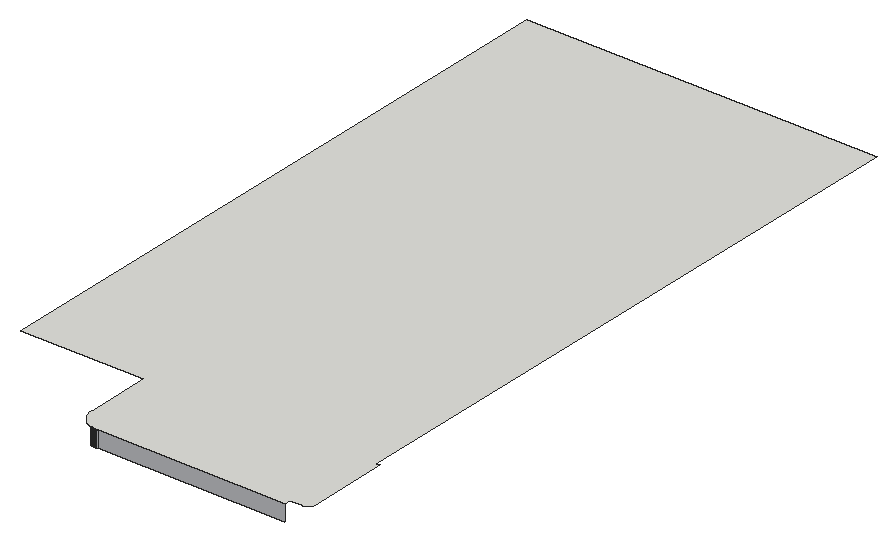
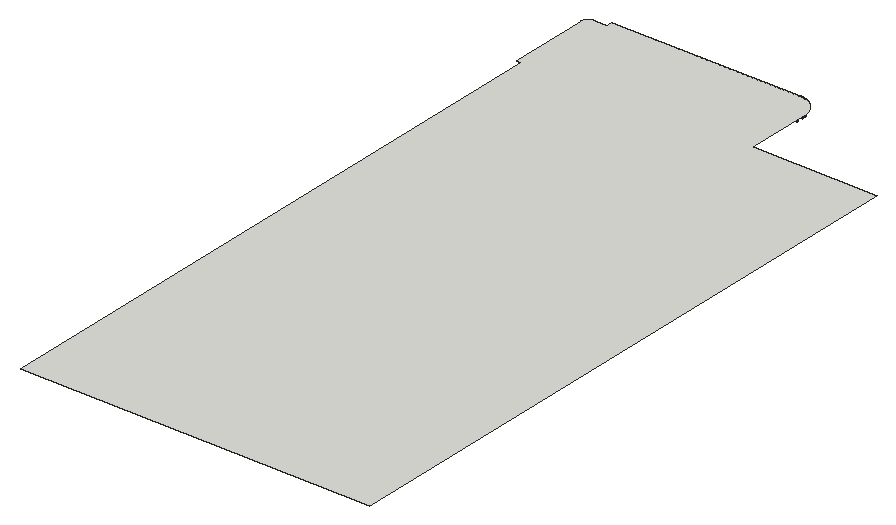
# SketchUp Ruby script. Lengths in inches.
U = 1.inch
M = Sketchup.active_model
def pt(a) = Geom::Point3d.new(a.map { |v| v * U })
def face(e, loops, mat)
  f = e.add_face(loops[0].map { |a| pt(a) })
  loops[1..].each { |l| e.add_face(l.map { |a| pt(a) }).erase! }
  f.material = f.back_material = mat if mat
  f
end
# faces: each face lists its corners as indices into pts; further lists are holes
def faces(e, pts, list, mat = nil) = list.each { |f| face(e, (f[0].is_a?(Array) ? f : [f]).map { |l| l.map { |i| pts[i] } }, mat) }
# xy, xz, yz: faces in a plane at the given z, y or x. An outline is a flat list of corners, or four numbers for a rectangle; further outlines are holes
def ring(l) = l.size == 4 ? [[l[0], l[1]], [l[2], l[1]], [l[2], l[3]], [l[0], l[3]]] : l.each_slice(2).to_a
def flat(e, list, mat, &to3) = list.each { |f| face(e, (f[0].is_a?(Array) ? f : [f]).map { |l| ring(l).map { |u, v| to3.(u, v) } }, mat) }
def xy(e, z, list, mat = nil) = flat(e, list, mat) { |x, y| [x, y, z] }
def xz(e, y, list, mat = nil) = flat(e, list, mat) { |x, z| [x, y, z] }
def yz(e, x, list, mat = nil) = flat(e, list, mat) { |y, z| [x, y, z] }
def lines(e, pts, list) = list.each { |a, b| e.add_line(pt(pts[a]), pt(pts[b])) }
# prism: a flat outline (further loops are holes) pulled along v
def prism(e, loops, v, mat = nil)
  f = face(e, loops, mat); d = Geom::Vector3d.new(v.map { |x| x * U })
  f.pushpull(f.normal.samedirection?(d) ? d.length : -d.length)
end
def box(e, o, s, mat = nil) = prism(e, [[o, [o[0] + s[0], o[1], o[2]], [o[0] + s[0], o[1] + s[1], o[2]], [o[0], o[1] + s[1], o[2]]]], [0, 0, s[2]], mat)
def at(x, y, z, deg = 0) = Geom::Transformation.translation(pt([x, y, z])) * Geom::Transformation.rotation(ORIGIN, Z_AXIS, deg.degrees)
def axes(o, x, y, z) = Geom::Transformation.new([*x, 0, *y, 0, *z, 0, *pt(o).to_a, 1])
def part(name) = M.definitions.add(name)
# library, detail: a bought-in or finely detailed component or shape, given as its bounding box
def library(name, o, s) = part(name).tap { |d| box(d.entities, o, s) }
def detail(e, o, s) = box(e.add_group.entities, o, s)
def put(e, d, t, mat = nil) = e.add_instance(d, t).tap { |i| i.material = mat if mat }
def group(e, t, mat = nil) = e.add_group.tap { |g| g.transformation = t; g.material = mat if mat }.entities
root = M.entities
M.materials.add("1427 AP 686 ARMOUR-N").color = [184, 186, 189]
xy(root,369,[[123.09,124,123.01,124.01,122.9375,124.02,122.86,124.03,122.78,124.04,122.7,124.06,122.63,124.08,122.55,124.1,122.48,124.12,122.4,124.15,122.26,124.21,122.1875,124.24,122.12,124.27,121.84,124.43,121.78,124.48,121.72,124.52,121.66,124.57,121.54,124.68,121.48,124.73,121.43,124.79,121.32,124.91,121.27,124.97,121.23,125.03,121.18,125.09,121.02,125.37,120.99,125.4375,120.96,125.51,120.9,125.65,120.87,125.73,120.85,125.8,120.83,125.88,120.81,125.95,120.79,126.03,120.78,126.11,120.77,126.1875,120.76,126.26,120.75,126.34,120.75,126.66,120.76,126.74,120.77,126.8125,120.78,126.89,120.79,126.97,120.81,127.05,120.83,127.12,120.85,127.2,120.87,127.27,120.9,127.35,120.96,127.49,120.99,127.5625,121.02,127.63,121.18,127.91,121.23,127.97,121.27,128.03,121.32,128.09,121.43,128.21,121.48,128.27,121.54,128.32,121.66,128.43,121.72,128.48,121.78,128.52,121.84,128.57,122.12,128.73,122.1875,128.76,122.26,128.79,122.4,128.85,122.48,128.88,122.55,128.9,122.63,128.92,122.7,128.94,122.78,128.96,122.86,128.97,122.9375,128.98,123.01,128.99,123.09,129,123.41,129,123.49,128.99,123.5625,128.98,123.64,128.97,123.72,128.96,123.8,128.94,123.87,128.92,123.95,128.9,124.02,128.88,124.1,128.85,124.24,128.79,124.3125,128.76,124.38,128.73,124.66,128.57,124.72,128.52,124.78,128.48,124.84,128.43,124.96,128.32,125.02,128.27,125.07,128.21,125.18,128.09,125.23,128.03,125.27,127.97,125.32,127.91,125.48,127.63,125.51,127.5625,125.54,127.49,125.6,127.35,125.63,127.27,125.65,127.2,125.67,127.12,125.69,127.05,125.71,126.97,125.72,126.89,125.73,126.8125,125.74,126.74,125.75,126.66,125.75,126.34,125.74,126.26,125.73,126.1875,125.72,126.11,125.71,126.03,125.69,125.95,125.67,125.88,125.65,125.8,125.63,125.73,125.6,125.65,125.54,125.51,125.51,125.4375,125.48,125.37,125.32,125.09,125.27,125.03,125.23,124.97,125.18,124.91,125.07,124.79,125.02,124.73,124.96,124.68,124.84,124.57,124.78,124.52,124.72,124.48,124.66,124.43,124.38,124.27,124.3125,124.24,124.24,124.21,124.1,124.15,124.02,124.12,123.95,124.1,123.87,124.08,123.8,124.06,123.72,124.04,123.64,124.03,123.5625,124.02,123.49,124.01,123.41,124],[186.97,124,186.89,124.01,186.8125,124.02,186.73,124.03,186.66,124.04,186.5,124.08,186.43,124.1,186.35,124.12,186.28,124.15,186.2,124.18,186.13,124.21,186.0625,124.24,185.99,124.27,185.85,124.35,185.79,124.39,185.72,124.43,185.66,124.48,185.59,124.52,185.53,124.57,185.41,124.68,185.3,124.79,185.1,125.03,185.06,125.09,185.01,125.16,184.93,125.3,184.9,125.37,184.86,125.4375,184.83,125.51,184.77,125.65,184.75,125.73,184.72,125.8,184.7,125.88,184.69,125.95,184.67,126.03,184.66,126.11,184.64,126.1875,184.64,126.26,184.63,126.34,184.625,126.42,184.625,126.58,184.63,126.66,184.64,126.74,184.64,126.8125,184.66,126.89,184.67,126.97,184.69,127.05,184.7,127.12,184.72,127.2,184.75,127.27,184.77,127.35,184.83,127.49,184.86,127.5625,184.9,127.63,184.93,127.7,185.01,127.84,185.06,127.91,185.1,127.97,185.3,128.21,185.41,128.32,185.53,128.43,185.59,128.48,185.66,128.52,185.72,128.57,185.79,128.61,185.85,128.65,185.99,128.73,186.0625,128.76,186.13,128.79,186.2,128.82,186.28,128.85,186.35,128.88,186.43,128.9,186.5,128.92,186.66,128.96,186.73,128.97,186.8125,128.98,186.89,128.99,186.97,129,187.28,129,187.36,128.99,187.4375,128.98,187.52,128.97,187.59,128.96,187.75,128.92,187.82,128.9,187.9,128.88,187.97,128.85,188.05,128.82,188.12,128.79,188.1875,128.76,188.26,128.73,188.4,128.65,188.46,128.61,188.53,128.57,188.59,128.52,188.66,128.48,188.72,128.43,188.84,128.32,188.95,128.21,189.15,127.97,189.19,127.91,189.24,127.84,189.32,127.7,189.35,127.63,189.39,127.5625,189.42,127.49,189.48,127.35,189.5,127.27,189.53,127.2,189.55,127.12,189.56,127.05,189.58,126.97,189.59,126.89,189.61,126.8125,189.61,126.74,189.62,126.66,189.625,126.58,189.625,126.42,189.62,126.34,189.61,126.26,189.61,126.1875,189.59,126.11,189.58,126.03,189.56,125.95,189.55,125.88,189.53,125.8,189.5,125.73,189.48,125.65,189.42,125.51,189.39,125.4375,189.35,125.37,189.32,125.3,189.24,125.16,189.19,125.09,189.15,125.03,188.95,124.79,188.84,124.68,188.72,124.57,188.66,124.52,188.59,124.48,188.53,124.43,188.46,124.39,188.4,124.35,188.26,124.27,188.1875,124.24,188.12,124.21,188.05,124.18,187.97,124.15,187.9,124.12,187.82,124.1,187.75,124.08,187.59,124.04,187.52,124.03,187.4375,124.02,187.36,124.01,187.28,124],[250.84,124,250.76,124.01,250.6875,124.02,250.61,124.03,250.53,124.04,250.45,124.06,250.38,124.08,250.3,124.1,250.23,124.12,250.15,124.15,249.94,124.24,249.86,124.27,249.8,124.31,249.59,124.43,249.53,124.48,249.47,124.52,249.41,124.57,249.29,124.68,249.23,124.73,249.18,124.79,249.07,124.91,249.02,124.97,248.98,125.03,248.93,125.09,248.77,125.37,248.74,125.4375,248.71,125.51,248.65,125.65,248.62,125.73,248.6,125.8,248.58,125.88,248.56,125.95,248.54,126.03,248.53,126.11,248.52,126.1875,248.51,126.26,248.5,126.34,248.5,126.66,248.51,126.74,248.52,126.8125,248.53,126.89,248.54,126.97,248.56,127.05,248.58,127.12,248.6,127.2,248.62,127.27,248.65,127.35,248.71,127.49,248.74,127.5625,248.77,127.63,248.93,127.91,248.98,127.97,249.02,128.03,249.07,128.09,249.18,128.21,249.23,128.27,249.29,128.32,249.41,128.43,249.47,128.48,249.53,128.52,249.59,128.57,249.8,128.69,249.86,128.73,249.94,128.76,250.15,128.85,250.23,128.88,250.3,128.9,250.38,128.92,250.45,128.94,250.53,128.96,250.61,128.97,250.6875,128.98,250.76,128.99,250.84,129,251.16,129,251.24,128.99,251.3125,128.98,251.39,128.97,251.47,128.96,251.55,128.94,251.62,128.92,251.7,128.9,251.77,128.88,251.85,128.85,251.99,128.79,252.0625,128.76,252.13,128.73,252.41,128.57,252.47,128.52,252.53,128.48,252.59,128.43,252.71,128.32,252.77,128.27,252.82,128.21,252.93,128.09,252.98,128.03,253.02,127.97,253.07,127.91,253.23,127.63,253.26,127.5625,253.29,127.49,253.35,127.35,253.38,127.27,253.4,127.2,253.42,127.12,253.44,127.05,253.46,126.97,253.47,126.89,253.48,126.8125,253.49,126.74,253.49,126.66,253.5,126.58,253.5,126.42,253.49,126.34,253.49,126.26,253.48,126.1875,253.47,126.11,253.46,126.03,253.44,125.95,253.42,125.88,253.4,125.8,253.38,125.73,253.35,125.65,253.29,125.51,253.26,125.4375,253.23,125.37,253.07,125.09,253.02,125.03,252.98,124.97,252.93,124.91,252.82,124.79,252.77,124.73,252.71,124.68,252.59,124.57,252.53,124.52,252.47,124.48,252.41,124.43,252.13,124.27,252.0625,124.24,251.99,124.21,251.85,124.15,251.77,124.12,251.7,124.1,251.62,124.08,251.55,124.06,251.47,124.04,251.39,124.03,251.3125,124.02,251.24,124.01,251.16,124],[123.09,170.25,123.01,170.26,122.9375,170.27,122.86,170.28,122.78,170.29,122.7,170.31,122.63,170.33,122.55,170.35,122.48,170.37,122.4,170.4,122.26,170.46,122.1875,170.49,122.12,170.52,121.84,170.68,121.78,170.73,121.72,170.77,121.66,170.82,121.54,170.93,121.48,170.98,121.43,171.04,121.32,171.16,121.27,171.22,121.23,171.28,121.18,171.34,121.02,171.62,120.99,171.6875,120.96,171.76,120.9,171.9,120.87,171.98,120.85,172.05,120.83,172.13,120.81,172.2,120.79,172.28,120.78,172.36,120.77,172.4375,120.76,172.51,120.75,172.59,120.75,172.91,120.76,172.99,120.77,173.0625,120.78,173.14,120.79,173.22,120.81,173.3,120.83,173.37,120.85,173.45,120.87,173.52,120.9,173.6,120.96,173.74,120.99,173.8125,121.02,173.88,121.18,174.16,121.23,174.22,121.27,174.28,121.32,174.34,121.43,174.46,121.48,174.52,121.54,174.57,121.66,174.68,121.72,174.73,121.78,174.77,121.84,174.82,122.12,174.98,122.1875,175.01,122.26,175.04,122.4,175.1,122.48,175.13,122.55,175.15,122.63,175.17,122.7,175.19,122.78,175.21,122.86,175.22,122.9375,175.23,123.01,175.24,123.09,175.25,123.41,175.25,123.49,175.24,123.5625,175.23,123.64,175.22,123.72,175.21,123.8,175.19,123.87,175.17,123.95,175.15,124.02,175.13,124.1,175.1,124.24,175.04,124.3125,175.01,124.38,174.98,124.66,174.82,124.72,174.77,124.78,174.73,124.84,174.68,124.96,174.57,125.02,174.52,125.07,174.46,125.18,174.34,125.23,174.28,125.27,174.22,125.32,174.16,125.48,173.88,125.51,173.8125,125.54,173.74,125.6,173.6,125.63,173.52,125.65,173.45,125.67,173.37,125.69,173.3,125.71,173.22,125.72,173.14,125.73,173.0625,125.74,172.99,125.75,172.91,125.75,172.59,125.74,172.51,125.73,172.4375,125.72,172.36,125.71,172.28,125.69,172.2,125.67,172.13,125.65,172.05,125.63,171.98,125.6,171.9,125.54,171.76,125.51,171.6875,125.48,171.62,125.32,171.34,125.27,171.28,125.23,171.22,125.18,171.16,125.07,171.04,125.02,170.98,124.96,170.93,124.84,170.82,124.78,170.77,124.72,170.73,124.66,170.68,124.38,170.52,124.3125,170.49,124.24,170.46,124.1,170.4,124.02,170.37,123.95,170.35,123.87,170.33,123.8,170.31,123.72,170.29,123.64,170.28,123.5625,170.27,123.49,170.26,123.41,170.25]])
xy(root,378,[[127.78,121,269,121,269,126,278.24,126,278.35,126.01,278.71,126.04,278.82,126.06,278.9375,126.07,279.05,126.09,279.17,126.12,279.29,126.14,279.4,126.17,279.51,126.19,279.63,126.23,279.85,126.29,279.97,126.33,280.08,126.37,280.1875,126.41,280.3,126.46,280.4,126.5,280.62,126.6,280.72,126.65,280.83,126.71,280.93,126.77,281.03,126.82,281.13,126.88,281.23,126.95,281.33,127.01,281.53,127.15,281.71,127.29,281.81,127.36,281.9,127.4375,281.99,127.51,282.07,127.59,282.16,127.67,282.24,127.76,282.33,127.84,282.41,127.93,282.48,128.01,282.5625,128.1,282.64,128.19,282.71,128.29,282.85,128.47,282.99,128.67,283.05,128.77,283.12,128.87,283.18,128.97,283.23,129.07,283.29,129.17,283.35,129.28,283.4,129.38,283.5,129.6,283.54,129.7,283.59,129.8125,283.63,129.92,283.67,130.03,283.71,130.15,283.77,130.37,283.81,130.49,283.83,130.6,283.86,130.71,283.88,130.83,283.91,130.95,283.93,131.0625,283.94,131.18,283.96,131.29,283.99,131.65,284,131.76,284,192,281,192,281,663,18,663,18,186,111,186,111,137.78,111.01,137.55,111.01,137.33,111.02,137.11,111.04,136.89,111.05,136.67,111.07,136.44,111.09,136.22,111.15,135.78,111.18,135.5625,111.21,135.34,111.25,135.12,111.28,134.9,111.33,134.68,111.37,134.47,111.47,134.03,111.52,133.82,111.58,133.6,111.64,133.39,111.7,133.17,111.76,132.96,111.9,132.54,111.98,132.33,112.05,132.12,112.29,131.49,112.47,131.09,112.5625,130.88,112.66,130.68,112.75,130.48,112.85,130.28,112.96,130.08,113.06,129.89,113.17,129.69,113.39,129.31,113.51,129.12,113.62,128.93,113.74,128.74,113.87,128.56,113.99,128.37,114.12,128.1875,114.25,128.01,114.51,127.65,114.65,127.48,114.79,127.3,115.07,126.96,115.22,126.79,115.52,126.46,115.82,126.14,116.14,125.82,116.46,125.52,116.79,125.22,116.96,125.07,117.3,124.79,117.48,124.65,117.65,124.51,118.01,124.25,118.1875,124.12,118.37,123.99,118.56,123.87,118.74,123.74,118.93,123.62,119.12,123.51,119.31,123.39,119.69,123.17,119.89,123.06,120.08,122.96,120.28,122.85,120.48,122.75,120.68,122.66,120.88,122.5625,121.09,122.47,121.49,122.29,122.12,122.05,122.33,121.98,122.54,121.9,122.96,121.76,123.17,121.7,123.39,121.64,123.6,121.58,123.82,121.52,124.03,121.47,124.47,121.37,124.68,121.33,124.9,121.28,125.12,121.25,125.34,121.21,125.5625,121.18,125.78,121.15,126.22,121.09,126.44,121.07,126.67,121.05,126.89,121.04,127.11,121.02,127.33,121.01,127.55,121.01]])
xz(root,121,[[127.78,366,128,378],[128,366,269,378]],"1427 AP 686 ARMOUR-N")
xz(root,121.01,[[127.33,366,127.55,378]],"1427 AP 686 ARMOUR-N")
xz(root,124,[[123.09,366,123.17,369],[123.17,366,123.25,369],[123.25,366,123.33,369],[123.33,366,123.41,369]])
xz(root,129,[[123.09,366,123.17,369],[123.17,366,123.25,369],[123.25,366,123.33,369],[123.33,366,123.41,369]])
xz(root,170.25,[[123.09,366,123.17,369],[123.17,366,123.25,369],[123.25,366,123.33,369],[123.33,366,123.41,369]])
yz(root,125.75,[[126.34,366,126.42,369],[126.42,366,126.5,369],[126.5,366,126.58,369],[126.58,366,126.66,369],[172.59,366,172.67,369],
  [172.67,366,172.75,369],[172.75,366,172.83,369],[172.83,366,172.91,369]])
p = [[126.67,121.05,366],[126.89,121.04,366],[126.89,121.04,378],[126.67,121.05,378],[127.11,121.02,366],[127.11,121.02,378],
  [127.33,121.01,366],[127.33,121.01,378],[127.55,121.01,366],[127.78,121,366],[127.78,121,378],[127.55,121.01,378],
  [125.5625,121.18,366],[125.78,121.15,366],[125.78,121.15,378],[125.5625,121.18,378],[126,121.12,366],[126,121.12,378],
  [126.22,121.09,366],[126.22,121.09,378],[126.44,121.07,366],[126.44,121.07,378],[124.9,121.28,366],[125.12,121.25,366],
  [125.12,121.25,378],[124.9,121.28,378],[125.34,121.21,366],[125.34,121.21,378],[124.47,121.37,366],[124.68,121.33,366],
  [124.68,121.33,378],[124.47,121.37,378],[124.03,121.47,366],[124.25,121.42,366],[124.25,121.42,378],[124.03,121.47,378],
  [123.6,121.58,366],[123.82,121.52,366],[123.82,121.52,378],[123.6,121.58,378],[123.17,121.7,366],[123.39,121.64,366],
  [123.39,121.64,378],[123.17,121.7,378],[122.96,121.76,366],[122.96,121.76,378],[122.54,121.9,366],[122.75,121.83,366],
  [122.75,121.83,378],[122.54,121.9,378],[122.78,124.04,366],[122.7,124.06,366],[122.7,124.06,369],[122.78,124.04,369],
  [122.86,124.03,366],[122.86,124.03,369],[122.9375,124.02,366],[122.9375,124.02,369],[123.01,124.01,366],[123.01,124.01,369],
  [123.09,124,366],[123.09,124,369],[123.49,124.01,366],[123.41,124,366],[123.41,124,369],[123.49,124.01,369],
  [123.5625,124.02,366],[123.5625,124.02,369],[123.64,124.03,366],[123.64,124.03,369],[123.72,124.04,366],[123.72,124.04,369],
  [123.8,124.06,366],[123.8,124.06,369],[122.63,124.08,366],[122.63,124.08,369],[123.87,124.08,366],[123.87,124.08,369],
  [123.95,124.1,366],[123.95,124.1,369],[124.02,124.12,366],[124.02,124.12,369],[124.1,124.15,366],[124.1,124.15,369],
  [124.17,124.18,366],[124.17,124.18,369],[124.24,124.21,366],[124.24,124.21,369],[124.3125,124.24,366],[124.3125,124.24,369],
  [124.38,124.27,366],[124.38,124.27,369],[124.45,124.31,366],[124.45,124.31,369],[124.52,124.35,366],[124.52,124.35,369],
  [124.59,124.39,366],[124.59,124.39,369],[124.66,124.43,366],[124.66,124.43,369],[124.72,124.48,366],[124.72,124.48,369],
  [124.78,124.52,366],[124.78,124.52,369],[124.84,124.57,366],[124.84,124.57,369],[124.9,124.625,366],[124.9,124.625,369],
  [124.96,124.68,366],[124.96,124.68,369],[125.02,124.73,366],[125.02,124.73,369],[125.07,124.79,366],[125.07,124.79,369],
  [125.125,124.85,366],[125.125,124.85,369],[125.18,124.91,366],[125.18,124.91,369],[125.23,124.97,366],[125.23,124.97,369],
  [125.27,125.03,366],[125.27,125.03,369],[125.32,125.09,366],[125.32,125.09,369],[125.36,125.16,366],[125.36,125.16,369],
  [125.4,125.23,366],[125.4,125.23,369],[125.44,125.3,366],[125.44,125.3,369],[125.48,125.37,366],[125.48,125.37,369],
  [125.51,125.4375,366],[125.51,125.4375,369],[125.54,125.51,366],[125.54,125.51,369],[125.57,125.58,366],[125.57,125.58,369],
  [125.6,125.65,366],[125.6,125.65,369],[125.63,125.73,366],[125.63,125.73,369],[125.65,125.8,366],[125.65,125.8,369],
  [125.67,125.88,366],[125.67,125.88,369],[125.69,125.95,366],[125.69,125.95,369],[125.71,126.03,366],[125.71,126.03,369],
  [125.72,126.11,366],[125.72,126.11,369],[125.73,126.1875,366],[125.73,126.1875,369],[125.74,126.26,366],[125.74,126.26,369],
  [125.75,126.34,366],[125.75,126.34,369],[125.73,126.8125,366],[125.74,126.74,366],[125.74,126.74,369],[125.73,126.8125,369],
  [125.75,126.66,366],[125.75,126.66,369],[125.72,126.89,366],[125.72,126.89,369],[125.71,126.97,366],[125.71,126.97,369],
  [125.67,127.12,366],[125.69,127.05,366],[125.69,127.05,369],[125.67,127.12,369],[125.65,127.2,366],[125.65,127.2,369],
  [125.63,127.27,366],[125.63,127.27,369],[125.57,127.42,366],[125.6,127.35,366],[125.6,127.35,369],[125.57,127.42,369],
  [125.54,127.49,366],[125.54,127.49,369],[125.51,127.5625,366],[125.51,127.5625,369],[125.44,127.7,366],[125.48,127.63,366],
  [125.48,127.63,369],[125.44,127.7,369],[125.4,127.77,366],[125.4,127.77,369],[125.32,127.91,366],[125.36,127.84,366],
  [125.36,127.84,369],[125.32,127.91,369],[125.27,127.97,366],[125.27,127.97,369],[125.18,128.09,366],[125.23,128.03,366],
  [125.23,128.03,369],[125.18,128.09,369],[125.125,128.15,366],[125.125,128.15,369],[125.02,128.27,366],[125.07,128.21,366],
  [125.07,128.21,369],[125.02,128.27,369],[124.9,128.375,366],[124.96,128.32,366],[124.96,128.32,369],[124.9,128.375,369],
  [124.78,128.48,366],[124.84,128.43,366],[124.84,128.43,369],[124.78,128.48,369],[124.66,128.57,366],[124.72,128.52,366],
  [124.72,128.52,369],[124.66,128.57,369],[124.52,128.65,366],[124.59,128.61,366],[124.59,128.61,369],[124.52,128.65,369],
  [124.3125,128.76,366],[124.38,128.73,366],[124.38,128.73,369],[124.3125,128.76,369],[124.45,128.69,366],[124.45,128.69,369],
  [124.1,128.85,366],[124.17,128.82,366],[124.17,128.82,369],[124.1,128.85,369],[124.24,128.79,366],[124.24,128.79,369],
  [122.55,128.9,366],[122.63,128.92,366],[122.63,128.92,369],[122.55,128.9,369],[122.7,128.94,366],[122.7,128.94,369],
  [122.78,128.96,366],[122.78,128.96,369],[123.72,128.96,366],[123.8,128.94,366],[123.8,128.94,369],[123.72,128.96,369],
  [123.87,128.92,366],[123.87,128.92,369],[123.95,128.9,366],[123.95,128.9,369],[124.02,128.88,366],[124.02,128.88,369],
  [122.86,128.97,366],[122.86,128.97,369],[122.9375,128.98,366],[122.9375,128.98,369],[123.01,128.99,366],[123.01,128.99,369],
  [123.09,129,366],[123.09,129,369],[123.41,129,366],[123.49,128.99,366],[123.49,128.99,369],[123.41,129,369],
  [123.5625,128.98,366],[123.5625,128.98,369],[123.64,128.97,366],[123.64,128.97,369],[122.63,170.33,366],[122.55,170.35,366],
  [122.55,170.35,369],[122.63,170.33,369],[122.7,170.31,366],[122.7,170.31,369],[122.78,170.29,366],[122.78,170.29,369],
  [122.86,170.28,366],[122.86,170.28,369],[122.9375,170.27,366],[122.9375,170.27,369],[123.01,170.26,366],[123.01,170.26,369],
  [123.09,170.25,366],[123.09,170.25,369],[123.49,170.26,366],[123.41,170.25,366],[123.41,170.25,369],[123.49,170.26,369],
  [123.5625,170.27,366],[123.5625,170.27,369],[123.64,170.28,366],[123.64,170.28,369],[123.72,170.29,366],[123.72,170.29,369],
  [123.8,170.31,366],[123.8,170.31,369],[123.87,170.33,366],[123.87,170.33,369],[123.95,170.35,366],[123.95,170.35,369],
  [124.02,170.37,366],[124.02,170.37,369],[124.1,170.4,366],[124.1,170.4,369],[124.17,170.43,366],[124.17,170.43,369],
  [124.24,170.46,366],[124.24,170.46,369],[124.3125,170.49,366],[124.3125,170.49,369],[124.38,170.52,366],[124.38,170.52,369],
  [124.45,170.56,366],[124.45,170.56,369],[124.52,170.6,366],[124.52,170.6,369],[124.59,170.64,366],[124.59,170.64,369],
  [124.66,170.68,366],[124.66,170.68,369],[124.72,170.73,366],[124.72,170.73,369],[124.78,170.77,366],[124.78,170.77,369],
  [124.84,170.82,366],[124.84,170.82,369],[124.9,170.875,366],[124.9,170.875,369],[124.96,170.93,366],[124.96,170.93,369],
  [125.02,170.98,366],[125.02,170.98,369],[125.07,171.04,366],[125.07,171.04,369],[125.125,171.1,366],[125.125,171.1,369],
  [125.18,171.16,366],[125.18,171.16,369],[125.23,171.22,366],[125.23,171.22,369],[125.27,171.28,366],[125.27,171.28,369],
  [125.32,171.34,366],[125.32,171.34,369],[125.36,171.41,366],[125.36,171.41,369],[125.4,171.48,366],[125.4,171.48,369],
  [125.44,171.55,366],[125.44,171.55,369],[125.48,171.62,366],[125.48,171.62,369],[125.51,171.6875,366],[125.51,171.6875,369],
  [125.54,171.76,366],[125.54,171.76,369],[125.57,171.83,366],[125.57,171.83,369],[125.6,171.9,366],[125.6,171.9,369],
  [125.63,171.98,366],[125.63,171.98,369],[125.65,172.05,366],[125.65,172.05,369],[125.67,172.13,366],[125.67,172.13,369],
  [125.69,172.2,366],[125.69,172.2,369],[125.71,172.28,366],[125.71,172.28,369],[125.72,172.36,366],[125.72,172.36,369],
  [125.73,172.4375,366],[125.73,172.4375,369],[125.74,172.51,366],[125.74,172.51,369],[125.75,172.59,366],[125.75,172.59,369],
  [125.74,172.99,366],[125.75,172.91,366],[125.75,172.91,369],[125.74,172.99,369],[125.73,173.0625,366],[125.73,173.0625,369],
  [125.71,173.22,366],[125.72,173.14,366],[125.72,173.14,369],[125.71,173.22,369],[125.69,173.3,366],[125.69,173.3,369],
  [125.67,173.37,366],[125.67,173.37,369],[125.63,173.52,366],[125.65,173.45,366],[125.65,173.45,369],[125.63,173.52,369],
  [125.6,173.6,366],[125.6,173.6,369],[125.57,173.67,366],[125.57,173.67,369],[125.51,173.8125,366],[125.54,173.74,366],
  [125.54,173.74,369],[125.51,173.8125,369],[125.48,173.88,366],[125.48,173.88,369],[125.44,173.95,366],[125.44,173.95,369],
  [125.36,174.09,366],[125.4,174.02,366],[125.4,174.02,369],[125.36,174.09,369],[125.32,174.16,366],[125.32,174.16,369],
  [125.23,174.28,366],[125.27,174.22,366],[125.27,174.22,369],[125.23,174.28,369],[125.125,174.4,366],[125.18,174.34,366],
  [125.18,174.34,369],[125.125,174.4,369],[125.07,174.46,366],[125.07,174.46,369],[125.02,174.52,366],[125.02,174.52,369]]
faces(root,p,[[0,1,2,3],[1,4,5,2],[4,6,7,5],[8,9,10,11],[12,13,14,15],[13,16,17,14],[16,18,19,17],[18,20,21,19],
  [20,0,3,21],[22,23,24,25],[23,26,27,24],[26,12,15,27],[28,29,30,31],[29,22,25,30],[32,33,34,35],[33,28,31,34],
  [36,37,38,39],[37,32,35,38],[40,41,42,43],[41,36,39,42],[44,40,43,45],[46,47,48,49],[47,44,45,48]],"1427 AP 686 ARMOUR-N")
faces(root,p,[[50,51,52,53],[54,50,53,55],[56,54,55,57],[58,56,57,59],[60,58,59,61],[62,63,64,65],[66,62,65,67],[68,66,67,69],
  [70,68,69,71],[72,70,71,73],[51,74,75,52],[76,72,73,77],[78,76,77,79],[80,78,79,81],[82,80,81,83],[84,82,83,85],
  [86,84,85,87],[88,86,87,89],[90,88,89,91],[92,90,91,93],[94,92,93,95],[96,94,95,97],[98,96,97,99],[100,98,99,101],
  [102,100,101,103],[104,102,103,105],[106,104,105,107],[108,106,107,109],[110,108,109,111],[112,110,111,113],[114,112,113,115],[116,114,115,117],
  [118,116,117,119],[120,118,119,121],[122,120,121,123],[124,122,123,125],[126,124,125,127],[128,126,127,129],[130,128,129,131],[132,130,131,133],
  [134,132,133,135],[136,134,135,137],[138,136,137,139],[140,138,139,141],[142,140,141,143],[144,142,143,145],[146,144,145,147],[148,146,147,149],
  [150,148,149,151],[152,150,151,153],[154,152,153,155],[156,154,155,157],[158,159,160,161],[159,162,163,160],[164,158,161,165],[166,164,165,167],
  [168,169,170,171],[169,166,167,170],[172,168,171,173],[174,172,173,175],[176,177,178,179],[177,174,175,178],[180,176,179,181],[182,180,181,183],
  [184,185,186,187],[185,182,183,186],[188,184,187,189],[190,191,192,193],[191,188,189,192],[194,190,193,195],[196,197,198,199],[197,194,195,198],
  [200,196,199,201],[202,203,204,205],[203,200,201,204],[206,207,208,209],[207,202,205,208],[210,211,212,213],[211,206,209,212],[214,215,216,217],
  [215,210,213,216],[218,219,220,221],[219,214,217,220],[222,223,224,225],[223,226,227,224],[226,218,221,227],[228,229,230,231],[229,232,233,230],
  [232,222,225,233],[234,235,236,237],[235,238,239,236],[238,240,241,239],[242,243,244,245],[243,246,247,244],[246,248,249,247],[248,250,251,249],
  [250,228,231,251],[240,252,253,241],[252,254,255,253],[254,256,257,255],[256,258,259,257],[260,261,262,263],[261,264,265,262],[264,266,267,265],
  [266,242,245,267],[268,269,270,271],[272,268,271,273],[274,272,273,275],[276,274,275,277],[278,276,277,279],[280,278,279,281],[282,280,281,283],
  [284,285,286,287],[288,284,287,289],[290,288,289,291],[292,290,291,293],[294,292,293,295],[296,294,295,297],[298,296,297,299],[300,298,299,301],
  [302,300,301,303],[304,302,303,305],[306,304,305,307],[308,306,307,309],[310,308,309,311],[312,310,311,313],[314,312,313,315],[316,314,315,317],
  [318,316,317,319],[320,318,319,321],[322,320,321,323],[324,322,323,325],[326,324,325,327],[328,326,327,329],[330,328,329,331],[332,330,331,333],
  [334,332,333,335],[336,334,335,337],[338,336,337,339],[340,338,339,341],[342,340,341,343],[344,342,343,345],[346,344,345,347],[348,346,347,349],
  [350,348,349,351],[352,350,351,353],[354,352,353,355],[356,354,355,357],[358,356,357,359],[360,358,359,361],[362,360,361,363],[364,362,363,365],
  [366,364,365,367],[368,366,367,369],[370,368,369,371],[372,370,371,373],[374,372,373,375],[376,374,375,377],[378,379,380,381],[382,378,381,383],
  [384,385,386,387],[385,382,383,386],[388,384,387,389],[390,388,389,391],[392,393,394,395],[393,390,391,394],[396,392,395,397],[398,396,397,399],
  [400,401,402,403],[401,398,399,402],[404,400,403,405],[406,404,405,407],[408,409,410,411],[409,406,407,410],[412,408,411,413],[414,415,416,417],
  [415,412,413,416],[418,419,420,421],[419,414,417,420],[422,418,421,423],[424,422,423,425]])
